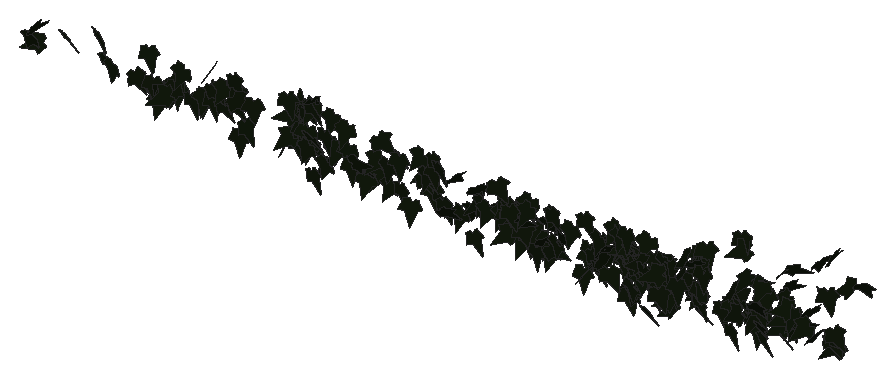
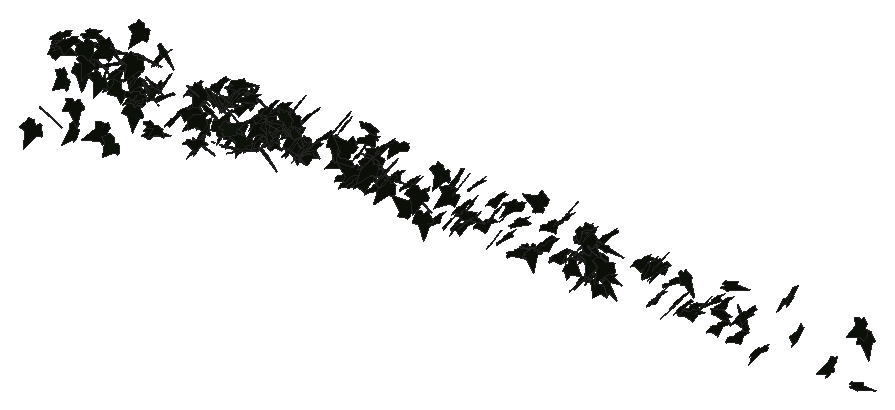
# SketchUp Ruby script. Lengths in inches.
U = 1.inch
M = Sketchup.active_model
def pt(a) = Geom::Point3d.new(a.map { |v| v * U })
def face(e, loops, mat)
  f = e.add_face(loops[0].map { |a| pt(a) })
  loops[1..].each { |l| e.add_face(l.map { |a| pt(a) }).erase! }
  f.material = f.back_material = mat if mat
  f
end
# faces: each face lists its corners as indices into pts; further lists are holes
def faces(e, pts, list, mat = nil) = list.each { |f| face(e, (f[0].is_a?(Array) ? f : [f]).map { |l| l.map { |i| pts[i] } }, mat) }
# xy, xz, yz: faces in a plane at the given z, y or x. An outline is a flat list of corners, or four numbers for a rectangle; further outlines are holes
def ring(l) = l.size == 4 ? [[l[0], l[1]], [l[2], l[1]], [l[2], l[3]], [l[0], l[3]]] : l.each_slice(2).to_a
def flat(e, list, mat, &to3) = list.each { |f| face(e, (f[0].is_a?(Array) ? f : [f]).map { |l| ring(l).map { |u, v| to3.(u, v) } }, mat) }
def xy(e, z, list, mat = nil) = flat(e, list, mat) { |x, y| [x, y, z] }
def xz(e, y, list, mat = nil) = flat(e, list, mat) { |x, z| [x, y, z] }
def yz(e, x, list, mat = nil) = flat(e, list, mat) { |y, z| [x, y, z] }
def lines(e, pts, list) = list.each { |a, b| e.add_line(pt(pts[a]), pt(pts[b])) }
# prism: a flat outline (further loops are holes) pulled along v
def prism(e, loops, v, mat = nil)
  f = face(e, loops, mat); d = Geom::Vector3d.new(v.map { |x| x * U })
  f.pushpull(f.normal.samedirection?(d) ? d.length : -d.length)
end
def box(e, o, s, mat = nil) = prism(e, [[o, [o[0] + s[0], o[1], o[2]], [o[0] + s[0], o[1] + s[1], o[2]], [o[0], o[1] + s[1], o[2]]]], [0, 0, s[2]], mat)
def at(x, y, z, deg = 0) = Geom::Transformation.translation(pt([x, y, z])) * Geom::Transformation.rotation(ORIGIN, Z_AXIS, deg.degrees)
def axes(o, x, y, z) = Geom::Transformation.new([*x, 0, *y, 0, *z, 0, *pt(o).to_a, 1])
def part(name) = M.definitions.add(name)
# library, detail: a bought-in or finely detailed component or shape, given as its bounding box
def library(name, o, s) = part(name).tap { |d| box(d.entities, o, s) }
def detail(e, o, s) = box(e.add_group.entities, o, s)
def put(e, d, t, mat = nil) = e.add_instance(d, t).tap { |i| i.material = mat if mat }
def group(e, t, mat = nil) = e.add_group.tap { |g| g.transformation = t; g.material = mat if mat }.entities
root = M.entities
M.materials.add("efeu1").color = [18, 25, 13]
c1 = part("ivyleaf_9")
p = [[1.54,2.16,1.25],[1.36,2.04,1.19],[-0.21,0.99,0.68],[-0.71,1.11,0.82],[-0.85,0.86,0.67],[-0.8,0.17,0.21],
  [-0.9,-0.01,0.1],[-0.67,-0.16,-0.02],[-0.08,-0.08,-0.05],[-0.03,-0.6,-0.4],[0.65,-0.88,-0.66],[0.83,-0.6,-0.49],
  [1.29,-0.42,-0.43],[1.8125,-0.07,-0.26],[1.21,0.44,0.15]]
faces(c1.entities,p,[[0,1,2,3,4,5,6,7,8,9,10,11,12,13,14]],"efeu1")
put(root,c1,axes([41.69,218.71,259.01],[0.16573,-0.44796,-0.14787],[-0.00628,0.15462,-0.47545],[0.47169,0.15945,0.04562]))
put(root,c1,axes([39.24,220.66,258.88],[-0.07317,-0.4717,0.14881],[-0.03935,-0.1444,-0.47707],[0.49305,-0.08153,-0.01599]))
put(root,c1,axes([54.97,220.37,258.9375],[0.15145,-0.468,-0.08964],[-0.03961,0.08137,-0.49174],[0.47486,0.15605,-0.01243]))
put(root,c1,axes([16.32,220.39,258.81],[-0.18161,-0.46555,0.01669],[-0.00257,-0.01691,-0.49971],[0.46584,-0.18159,0.00375]))
put(root,c1,axes([22.93,219.74,258.84],[0.01164,-0.49829,0.03967],[0.00611,-0.03954,-0.4984],[0.49983,0.01209,0.00516]))
put(root,c1,axes([39.71,221.03,259.17],[0.32737,0.18521,-0.32943],[-0.29143,-0.15376,-0.37607],[-0.24061,0.43824,0.00728]))
put(root,c1,axes([32.42,220.2,259.08],[-0.36225,-0.30732,-0.15597],[0.1342,0.08264,-0.47451],[0.31743,-0.38565,0.02261]))
put(root,c1,axes([29.26,220.11,259.07],[-0.14548,0.17352,-0.44579],[0.24229,-0.37503,-0.22505],[-0.41247,-0.2815,0.02503]))
put(root,c1,axes([61.79,221.22,258.85],[0.05915,0.49649,0.00142],[-0.00255,0.00173,-0.49999],[-0.49648,0.05915,0.00274]))
put(root,c1,axes([13.71,221.22,259.1875],[0.14882,-0.40431,-0.25374],[-0.02746,0.25809,-0.42736],[0.47655,0.14113,0.05461]))
put(root,c1,axes([26.28,221.05,259.14],[-0.25408,-0.11462,-0.4151],[0.37181,0.18476,-0.27861],[0.21726,-0.45025,-0.00866]))
put(root,c1,axes([32.18,220.24,259.23],[0.29071,0.15833,-0.37473],[-0.31652,-0.20129,-0.3306],[-0.25554,0.42944,-0.0168]))
put(root,c1,axes([62.04,220.71,258.93],[-0.07555,-0.49374,0.02259],[-0.00396,-0.02225,-0.49949],[0.49424,-0.07565,-0.00055]))
put(root,c1,axes([36.5,219.28,259.08],[-0.15881,-0.46494,-0.0928],[0.04255,0.08349,-0.49114],[0.4722,-0.16389,0.01305]))
put(root,c1,axes([52.36,220.61,258.96],[-0.42761,0.25803,-0.02383],[0.02061,-0.01196,-0.49943],[-0.25831,-0.42811,-0.00041]))
put(root,c1,axes([62.79,219.9,258.9375],[0.35697,-0.35001,-0.00792],[-0.00575,0.00545,-0.49994],[0.35005,0.35702,-0.00013]))
put(root,c1,axes([44.42,220.125,259.06],[-0.13816,-0.46076,0.13643],[-0.02366,-0.13526,-0.48078],[0.47995,-0.1393,0.01557]))
put(root,c1,axes([25.93,220.79,259.3],[-0.36566,0.2183,-0.26199],[0.20922,-0.15974,-0.4251],[-0.2693,-0.42051,0.02548]))
put(root,c1,axes([27.32,221.23,259.16],[0.30537,-0.38504,-0.09217],[0.01165,0.12509,-0.48396],[0.39574,0.29342,0.08537]))
put(root,c1,axes([54.62,219.83,259.08],[0.18919,-0.4047,0.22455],[0.1068,-0.19787,-0.44659],[0.45033,0.21695,0.01158]))
put(root,c1,axes([6.75,220.89,258.99],[-0.38467,-0.03692,0.25686],[-0.25164,-0.10565,-0.36589],[0.09703,-0.42036,0.0694]))
put(root,c1,axes([34.71,220.43,259.08],[0.2028,-0.45648,0.02225],[0.00841,-0.02061,-0.4995],[0.45695,0.20297,-0.00069]))
put(root,c1,axes([58.93,221,259.14],[0.08504,-0.49088,-0.04243],[-0.00119,0.04285,-0.49816],[0.49271,0.08483,0.00612]))
put(root,c1,axes([38.07,220.35,259.25],[0.19269,-0.4498,-0.10273],[-0.01302,0.10598,-0.48847],[0.4612,0.19092,0.02913]))
put(root,c1,axes([46.64,220.1,259.11],[-0.18728,-0.46245,0.03264],[-0.00218,-0.03432,-0.49882],[0.4636,-0.18698,0.01083]))
put(root,c1,axes([34.23,220.23,259.19],[-0.14658,-0.42022,0.22788],[-0.02607,-0.23097,-0.44269],[0.47732,-0.14166,0.0458]))
put(root,c1,axes([52.9,221.55,259.33],[0.24652,-0.36119,-0.24243],[0.20815,0.34262,-0.2988],[0.38197,0.04639,0.31929]))
put(root,c1,axes([53.79,218.56,259.38],[-0.02969,-0.46767,-0.17437],[0.04877,0.17112,-0.46727],[0.49673,-0.04475,0.03545]))
put(root,c1,axes([53.83,218.93,259.17],[-0.04068,-0.3651,0.33919],[0.10105,-0.33929,-0.35309],[0.48799,0.03982,0.10139]))
put(root,c1,axes([57.86,219.92,259.12],[0.48604,-0.11731,-0.00069],[-0.00037,0.00138,-0.5],[0.11731,0.48604,0.00125]))
put(root,c1,axes([32.71,221.06,259.17],[-0.31043,-0.38829,0.05349],[-0.0165,-0.05522,-0.49667],[0.39161,-0.31013,0.02147]))
put(root,c1,axes([29.59,219.73,259.24],[-0.09074,-0.41676,0.26091],[0.07648,-0.27405,-0.41115],[0.48571,-0.03471,0.11349]))
put(root,c1,axes([37.37,220.73,259.23],[0.21803,-0.43203,0.12574],[0.04934,-0.11592,-0.48387],[0.44724,0.22341,-0.00792]))
put(root,c1,axes([62.04,220.3,259.33],[0.4857,0.0514,-0.10701],[-0.10775,0.00161,-0.48825],[-0.04985,0.49735,0.01264]))
put(root,c1,axes([62.48,225.95,259.27],[0.47019,-0.16105,-0.0546],[-0.0544,0.00964,-0.49694],[0.16111,0.47326,-0.00846]))
put(root,c1,axes([53.09,220.74,259.22],[-0.10975,-0.48643,0.03663],[0.00253,-0.03811,-0.49854],[0.4878,-0.10924,0.01083]))
put(root,c1,axes([49.95,218.98,259.3125],[-0.02277,-0.4978,-0.0409],[-0.00504,0.04117,-0.49828],[0.49946,-0.02228,-0.0069]))
put(root,c1,axes([54.66,220.68,259.48],[-0.11745,-0.19356,-0.44581],[0.42836,0.17543,-0.18902],[0.22959,-0.42633,0.12462]))
put(root,c1,axes([45.78,220.8,259.31],[-0.12054,-0.481,0.06407],[-0.01894,-0.06131,-0.49587],[0.48488,-0.12197,-0.00344]))
put(root,c1,axes([53.82,220.59,259.36],[0.26998,0.41269,0.08248],[-0.12056,0.16973,-0.45459],[-0.40321,0.22557,0.19116]))
put(root,c1,axes([50.375,219.18,259.65],[-0.32192,0.25455,-0.2856],[0.12611,-0.2818,-0.3933],[-0.3612,-0.32526,0.11724]))
put(root,c1,axes([29.81,218.08,259.39],[0.23594,-0.43705,-0.05764],[-0.01788,0.05583,-0.49655],[0.44047,0.23637,0.01071]))
put(root,c1,axes([44.86,220.33,259.43],[-0.10661,-0.48137,-0.08319],[0.01205,0.08253,-0.49299],[0.48835,-0.10712,-0.006]))
put(root,c1,axes([59.57,226,259.39],[0.17712,0.35875,0.29987],[0.0105,0.31754,-0.38608],[-0.46746,0.14306,0.10495]))
put(root,c1,axes([27.34,220.94,259.375],[-0.08938,-0.48796,0.06251],[-0.00694,-0.06228,-0.49606],[0.4919,-0.08954,0.00435]))
put(root,c1,axes([56.33,220.95,259.5],[0.37584,-0.31786,-0.08783],[-0.07859,0.043,-0.49191],[0.32027,0.38356,-0.01764]))
put(root,c1,axes([54.625,220.75,259.67],[-0.35385,-0.25883,-0.24042],[0.20642,0.12466,-0.43801],[0.28668,-0.40923,0.01864]))
put(root,c1,axes([36.77,220.95,259.59],[-0.04253,-0.48051,-0.13152],[0.03312,0.12898,-0.48194],[0.49709,-0.04971,0.02086]))
put(root,c1,axes([64.37,227.57,259.56],[0.4073,0.27528,-0.09128],[-0.08776,-0.033,-0.49113],[-0.27642,0.41609,0.02143]))
put(root,c1,axes([45.16,220.92,259.51],[-0.23171,-0.38991,0.21044],[-0.06106,-0.20711,-0.45097],[0.43884,-0.23468,0.04837]))
put(root,c1,axes([20.5,220.95,259.66],[0.28001,-0.38775,-0.14576],[-0.00496,0.17278,-0.46917],[0.41421,0.26419,0.09292]))
put(root,c1,axes([49.34,220.45,259.64],[-0.26201,-0.40743,-0.1239],[0.13422,0.05906,-0.47801],[0.40415,-0.28375,0.07842]))
put(root,c1,axes([17.14,221.1,259.55],[-0.09752,-0.48565,-0.0681],[0.00461,0.06852,-0.49526],[0.49038,-0.09722,-0.00889]))
put(root,c1,axes([57.49,220.74,259.66],[0.0164,0.23513,-0.44096],[-0.30455,-0.34509,-0.19534],[-0.3962,0.275,0.1319]))
put(root,c1,axes([44,219.45,259.625],[-0.46706,-0.11291,0.13822],[-0.10279,-0.14639,-0.46691],[0.1459,-0.46457,0.11353]))
put(root,c1,axes([26.22,220.63,259.61],[-0.43913,-0.20773,0.11838],[-0.10836,-0.04776,-0.48577],[0.21313,-0.45229,-0.00307]))
put(root,c1,axes([19.25,221.02,259.75],[-0.23563,-0.42311,-0.12434],[0.10442,0.08344,-0.4818],[0.42846,-0.25302,0.04904]))
put(root,c1,axes([55.14,223.41,259.82],[0.32334,-0.33409,-0.18395],[-0.1165,0.14312,-0.4647],[0.36315,0.34337,0.0147]))
put(root,c1,axes([53.73,218.85,259.6875],[0.03024,-0.43514,0.24441],[0.13468,-0.22866,-0.42376],[0.48057,0.09146,0.10339]))
put(root,c1,axes([61.77,220.61,259.67],[-0.12781,-0.43897,0.20241],[-0.01881,-0.20469,-0.45579],[0.48302,-0.12413,0.03581]))
put(root,c1,axes([40.8125,220.99,259.07],[-0.02306,-0.1513,0.476],[0.48172,0.11917,0.06122],[-0.13198,0.46142,0.14027]))
put(root,c1,axes([57.32,218.41,259.64],[-0.43004,0.24718,0.06301],[-0.06249,0.01766,-0.49577],[-0.24731,-0.43427,0.0157]))
put(root,c1,axes([61.49,218.55,259.6],[0.26354,-0.42484,-0.00764],[-0.00427,0.00634,-0.49994],[0.42489,0.26357,-0.00028]))
put(root,c1,axes([55.35,223.22,259.73],[-0.49372,0.05722,-0.05448],[0.03949,-0.11994,-0.48379],[-0.06843,-0.48202,0.11392]))
put(root,c1,axes([55.05,223.31,259.67],[0.34376,-0.36173,-0.03131],[-0.02145,0.02281,-0.49902],[0.36245,0.34443,0.00016]))
put(root,c1,axes([63.98,219.98,259.63],[0.47281,-0.16259,0.00317],[0.00295,-0.00116,-0.49999],[0.1626,0.47282,-0.00013]))
put(root,c1,axes([61.97,221.16,259.81],[-0.40378,-0.27697,-0.10123],[0.09063,0.04678,-0.48949],[0.28062,-0.41364,0.01243]))
put(root,c1,axes([26.39,221.14,259.87],[0.18887,-0.44638,-0.12277],[0.03426,0.14571,-0.47707],[0.46169,0.1718,0.08563]))
put(root,c1,axes([50.34,220.68,259.75],[-0.49796,-0.01225,-0.04345],[0.04452,-0.05357,-0.49512],[0.00748,-0.49697,0.05444]))
put(root,c1,axes([58.09,219.83,259.73],[0.22386,-0.43493,0.10354],[0.07699,-0.07657,-0.48807],[0.44041,0.23446,0.03269]))
put(root,c1,axes([50.67,219.66,259.94],[0.07987,0.45465,-0.19212],[-0.01344,-0.19254,-0.46124],[-0.4934,0.07884,-0.01854]))
put(root,c1,axes([44.51,219.96,259.99],[-0.06521,-0.42857,-0.24915],[0.08718,0.23747,-0.43129],[0.488,-0.09969,0.04375]))
put(root,c1,axes([56.15,216.97,259.72],[0.4921,-0.08064,-0.03659],[-0.03581,0.00769,-0.49866],[0.08098,0.49339,0.00179]))
put(root,c1,axes([49.64,220.14,259.96],[0.24301,-0.38787,-0.20126],[-0.06196,0.19738,-0.4552],[0.43256,0.24617,0.04787]))
put(root,c1,axes([64.68,220.83,259.78],[0.10046,0.44382,0.2072],[-0.00703,0.21279,-0.4524],[-0.48975,0.08798,0.04899]))
put(root,c1,axes([66.26,220.6,259.74],[0.00095,0.49427,0.07544],[-0.02655,0.07539,-0.49357],[-0.49929,-0.00307,0.02639]))
put(root,c1,axes([39.33,218.67,259.78],[0.43694,0.19508,0.14501],[0.12825,0.06837,-0.47841],[-0.20649,0.45527,0.00971]))
put(root,c1,axes([51.6,220.92,260.0625],[-0.29164,-0.26929,-0.30402],[0.31034,0.09366,-0.38068],[0.26198,-0.41074,0.11251]))
put(root,c1,axes([45.79,219.95,259.22],[0.23112,0.43493,-0.08614],[0.03892,0.07686,0.49252],[0.44167,-0.23437,0.00167]))
put(root,c1,axes([31.37,219.88,259.79],[0.01229,-0.49841,-0.03791],[-0.01208,0.03761,-0.49844],[0.4997,0.01317,-0.01112]))
put(root,c1,axes([19.9,220.87,259.83],[0.07931,-0.4908,-0.05311],[0.00582,0.05471,-0.49696],[0.49364,0.07821,0.01439]))
put(root,c1,axes([52.03,218.82,260.1],[-0.09216,-0.34578,-0.3492],[0.25334,0.27101,-0.33522],[0.4211,-0.23872,0.12525]))
put(root,c1,axes([52.65,220.52,259.99],[0.19306,-0.42504,-0.17909],[-0.07474,0.16274,-0.46683],[0.45513,0.20702,-0.0007]))
put(root,c1,axes([55.03,220.82,260.07],[0.41335,-0.12484,-0.2521],[-0.23994,0.07744,-0.43178],[0.14685,0.47793,0.00411]))
put(root,c1,axes([16.01,219.78,259.26],[-0.06461,0.13814,0.47618],[0.21119,-0.4268,0.15247],[0.44858,0.22082,-0.0032]))
put(root,c1,axes([28.2,219.74,259.89],[-0.1261,-0.42195,0.23677],[0.03539,-0.25207,-0.43036],[0.48254,-0.09177,0.09344]))
put(root,c1,axes([64.54,220.8,259.7],[0.21885,-0.16164,-0.41949],[0.3376,-0.249,0.27208],[-0.29687,-0.40233,0.00015]))
put(root,c1,axes([57.28,218.625,259.81],[-0.37005,-0.02777,0.3351],[-0.33428,-0.02356,-0.37109],[0.0364,-0.49867,-0.00113]))
put(root,c1,axes([60.1875,225.96,259.87],[0.37223,0.12545,0.30937],[0.27404,0.14981,-0.39046],[-0.19066,0.46024,0.04277]))
put(root,c1,axes([47.0625,219.36,259.72],[0.02745,-0.04723,-0.49701],[0.25411,0.42978,-0.02681],[0.42974,-0.25112,0.0476]))
put(root,c1,axes([29.61,220.83,259.87],[-0.20986,-0.45033,0.0562],[-0.01511,-0.05496,-0.49674],[0.45357,-0.21019,0.00946]))
put(root,c1,axes([50.8,219.12,259.88],[0.30972,-0.38753,0.06243],[0.04191,-0.04642,-0.49607],[0.39028,0.31252,0.00372]))
put(root,c1,axes([46.73,218.42,259.9],[0.09436,-0.48341,0.08611],[0.00691,-0.08637,-0.49243],[0.49097,0.09412,-0.00962]))
put(root,c1,axes([53.77,221.72,259.18],[0.4983,-0.0009,-0.04115],[0.0028,0.49946,0.02305],[0.04107,-0.0232,0.49777]))
put(root,c1,axes([64.3,220.29,259.88],[-0.26768,-0.21714,0.36221],[-0.16084,-0.34411,-0.32515],[0.39049,-0.29058,0.11437]))
put(root,c1,axes([36.2,220.7,260.14],[0.2277,-0.41442,-0.16251],[0.04668,0.20377,-0.4542],[0.44269,0.19167,0.13149]))
put(root,c1,axes([60.08,220.6,260.07],[-0.0337,-0.48837,-0.1018],[0.16746,0.08504,-0.46339],[0.46992,-0.06532,0.15783]))
put(root,c1,axes([19.41,220.86,259.89],[-0.16168,-0.47281,0.01758],[0.00196,-0.01925,-0.49963],[0.47313,-0.16149,0.00807]))
put(root,c1,axes([8.19,221.2,259.95],[0.39839,-0.28631,0.09649],[0.09239,-0.03658,-0.49003],[0.28766,0.40828,0.02376]))
put(root,c1,axes([63.02,221.01,259.71],[-0.20239,0.32814,-0.31837],[-0.16632,0.27147,0.38554],[0.42588,0.26196,-0.00073]))
put(root,c1,axes([18.95,220.03,259.93],[0.17931,-0.46594,-0.02736],[-0.00666,0.02675,-0.49924],[0.46669,0.1794,0.00339]))
put(root,c1,axes([21.58,220.74,260.17],[0.3021,-0.35458,-0.18168],[-0.0486,0.1935,-0.45847],[0.39544,0.29467,0.08245]))
put(root,c1,axes([64.5625,226.38,260],[-0.40796,0.24106,0.15954],[-0.16255,0.03689,-0.4714],[-0.23905,-0.43649,0.04827]))
put(root,c1,axes([16.05,220.02,260.04],[-0.03343,-0.49333,-0.07424],[0.04361,0.07123,-0.49297],[0.49697,-0.03944,0.03827]))
put(root,c1,axes([49.15,220.48,260.01],[0.10157,-0.47537,0.11709],[0.02379,-0.11465,-0.4861],[0.489,0.10432,-0.00067]))
put(root,c1,axes([54.98,224,260.24],[-0.24806,-0.39153,-0.18753],[0.15276,0.12345,-0.45981],[0.40636,-0.28542,0.05837]))
put(root,c1,axes([61.7,220.19,260.07],[-0.40651,0.28662,-0.05099],[0.04639,-0.02269,-0.49733],[-0.2874,-0.40907,-0.00815]))
put(root,c1,axes([42.78,220.54,260.02],[0.45585,0.20495,-0.01394],[-0.0132,-0.00465,-0.4998],[-0.205,0.45604,0.00117]))
put(root,c1,axes([47.375,219.625,260.12],[0.03099,-0.42769,0.25714],[0.08492,-0.24935,-0.42498],[0.49176,0.07002,0.05718]))
put(root,c1,axes([29.41,220.93,260.09],[-0.10067,-0.48783,-0.04342],[0.00299,0.04371,-0.49808],[0.48975,-0.10054,-0.00588]))
put(root,c1,axes([57.97,220.22,260.14],[-0.19334,-0.40555,0.21943],[-0.05572,-0.21564,-0.44765],[0.45773,-0.19755,0.03819]))
put(root,c1,axes([17.52,220.52,260.15],[-0.46793,-0.16429,-0.06364],[0.05728,0.02891,-0.49587],[0.16661,-0.47135,-0.00824]))
put(root,c1,axes([40.67,220.59,260.09],[-0.47129,0.16676,-0.0086],[0.00526,-0.01092,-0.49985],[-0.1669,-0.47125,0.00853]))
put(root,c1,axes([51.83,220.65,260.125],[-0.02083,-0.49478,0.06899],[-0.00624,-0.06879,-0.49521],[0.49953,-0.0215,-0.0033]))
put(root,c1,axes([51.68,220.59,260.26],[0.41021,-0.27013,-0.09357],[-0.05755,0.08227,-0.48982],[0.28002,0.41263,0.0364]))
put(root,c1,axes([60.48,220.84,260.21],[0.16317,-0.39212,0.26386],[0.20734,-0.19146,-0.41274],[0.42472,0.24411,0.10012]))
put(root,c1,axes([51.87,220.72,260.43],[-0.39124,-0.14506,-0.27548],[0.26218,0.08508,-0.41716],[0.16791,-0.47087,0.00949]))
put(root,c1,axes([24.09,218.8125,260.4],[0.15106,-0.43018,-0.20525],[-0.05931,0.19668,-0.45585],[0.47293,0.16207,0.00839]))
put(root,c1,axes([62.14,220.65,260.5],[-0.1874,-0.32625,-0.3293],[0.23879,0.2365,-0.3702],[0.39732,-0.29602,0.06717]))
put(root,c1,axes([41.72,220.11,260.25],[-0.12547,-0.45523,0.16438],[-0.01502,-0.16607,-0.47138],[0.48377,-0.12323,0.028]))
put(root,c1,axes([42.92,220.35,260.2],[-0.01585,-0.49946,-0.01711],[-0.01839,0.01769,-0.49935],[0.49941,-0.0152,-0.01893]))
put(root,c1,axes([26.71,220.95,260.23],[0.02157,-0.49923,-0.01738],[-0.00001,0.01739,-0.4997],[0.49953,0.02156,0.00074]))
put(root,c1,axes([30.59,220.68,260.23],[-0.06932,-0.49413,0.03215],[-0.00061,-0.03238,-0.49895],[0.49517,-0.06922,0.00389]))
put(root,c1,axes([41.18,220.27,260.31],[-0.09723,-0.38036,0.30963],[0.04521,-0.32126,-0.38046],[0.48837,-0.04599,0.09687]))
put(root,c1,axes([17.79,219.88,260.3125],[-0.07559,-0.48802,0.07822],[-0.02242,-0.07566,-0.49373],[0.49374,-0.07815,-0.01044]))
put(root,c1,axes([27.84,220.15,260.37],[0.34932,-0.34476,0.09546],[0.14109,0.01017,-0.47957],[0.32874,0.36199,0.10439]))
put(root,c1,axes([57.79,220.3,260.3],[0.02981,-0.49825,0.02928],[-0.00586,-0.02968,-0.49908],[0.49908,0.02942,-0.00761]))
put(root,c1,axes([19.86,220.84,260.6],[0.26088,-0.36655,-0.21813],[-0.02031,0.24473,-0.43554],[0.42606,0.23611,0.1128]))
put(root,c1,axes([42.82,220.22,260.41],[-0.16322,-0.46023,0.10746],[-0.02535,-0.105,-0.48819],[0.47193,-0.16482,0.01094]))
put(root,c1,axes([68.67,220.11,260.21],[-0.0373,-0.01631,-0.49834],[-0.04251,-0.49781,0.01947],[-0.49679,0.04383,0.03575]))
put(root,c1,axes([65.94,220.17,260.41],[0.22563,0.44222,0.05942],[0.03132,0.05073,-0.49643],[-0.44509,0.22775,-0.00481]))
put(root,c1,axes([51.51,219.33,260.1],[-0.38339,0.21841,-0.23517],[-0.20376,0.11742,0.44124],[0.24797,0.43418,-0.00103]))
put(root,c1,axes([68.2,220,260.71],[0.05281,-0.42555,-0.25714],[0.04577,0.26164,-0.42361],[0.49509,0.0212,0.06659]))
put(root,c1,axes([56.57,217.88,260.72],[-0.15218,-0.33177,-0.34171],[0.2058,0.27771,-0.36128],[0.42952,-0.25061,0.05203]))
put(root,c1,axes([36.45,221.19,260.46],[-0.44486,-0.14425,0.1769],[-0.1682,-0.05481,-0.46766],[0.15432,-0.47559,0.00024]))
put(root,c1,axes([27.6,220.42,260.56],[-0.20618,-0.44594,-0.09289],[0.1083,0.05105,-0.48545],[0.44245,-0.2203,0.07554]))
put(root,c1,axes([56.83,220.62,260.4375],[-0.4958,0.06197,0.01858],[-0.01939,-0.00531,-0.4996],[-0.06173,-0.49612,0.00767]))
put(root,c1,axes([49.62,221.19,260.51],[0.30168,-0.39805,-0.02331],[-0.00013,0.02913,-0.49915],[0.39874,0.30117,0.01747]))
put(root,c1,axes([64.49,220.42,260.58],[-0.40414,-0.15086,0.25281],[-0.1434,-0.27411,-0.39281],[0.25711,-0.39,0.1783]))
put(root,c1,axes([50.92,221.04,260.67],[0.35232,-0.34508,-0.08239],[0.02418,0.1392,-0.47962],[0.35395,0.33398,0.11477]))
put(root,c1,axes([57.4375,225.39,260.5625],[-0.37642,-0.1329,0.30107],[-0.26903,-0.13919,-0.39781],[0.18955,-0.46148,0.03328]))
put(root,c1,axes([53.17,220.02,260.83],[0.03272,-0.42127,-0.26733],[-0.02806,0.26592,-0.42249],[0.49814,0.04265,-0.00623]))
put(root,c1,axes([18.59,218.34,260.62],[-0.40367,-0.13443,0.26263],[-0.2316,-0.13136,-0.42321],[0.18279,-0.46333,0.04379]))
put(root,c1,axes([33.22,220.28,260.65],[-0.2737,-0.37267,0.19028],[-0.07164,-0.18228,-0.46005],[0.41226,-0.27909,0.04638]))
put(root,c1,axes([44.68,219.13,260.63],[0.3405,0.25433,0.26339],[0.20641,0.16375,-0.42495],[-0.30241,0.39813,0.00652]))
put(root,c1,axes([34.21,219.87,260.6875],[0.0084,-0.44565,0.22655],[0.0696,-0.22333,-0.4419],[0.49506,0.03896,0.05829]))
put(root,c1,axes([36.63,220.5625,260.67],[0.01287,-0.44347,0.23059],[-0.00469,-0.23077,-0.44354],[0.49981,0.00926,-0.0101]))
put(root,c1,axes([40.13,220.92,260.65],[0.2468,0.43254,-0.04474],[-0.01994,-0.04013,-0.49799],[-0.43439,0.24759,-0.00256]))
put(root,c1,axes([51.96,220.375,260.68],[-0.02057,0.47814,0.14476],[-0.03846,0.14294,-0.47759],[-0.49809,-0.03078,0.0309]))
put(root,c1,axes([47.92,219.375,260.87],[0.26375,0.0668,-0.41949],[-0.4184,-0.04438,-0.27013],[-0.07333,0.49353,0.03249]))
put(root,c1,axes([51.21,218.93,260.52],[0.00466,0.09511,-0.49085],[-0.21308,0.44444,0.08409],[0.4523,0.20839,0.04468]))
put(root,c1,axes([7.83,218.39,260.94],[0.28455,0.13928,-0.38682],[-0.36268,-0.13651,-0.31595],[-0.19363,0.4604,0.02334]))
put(root,c1,axes([55.84,218.97,260.65],[0.04123,-0.49788,0.02032],[0.00326,-0.02012,-0.49958],[0.49829,0.04132,0.00159]))
put(root,c1,axes([65.2,220.55,260.76],[-0.48215,0.11354,-0.06813],[0.0612,-0.03706,-0.49486],[-0.11742,-0.48553,0.02184]))
put(root,c1,axes([54.9375,221.78,260.1],[-0.45794,-0.08004,0.18407],[0.10732,-0.48512,0.05606],[0.16962,0.09086,0.46149]))
put(root,c1,axes([25.74,220.83,260.73],[0.33446,0.36565,0.06664],[0.03702,0.05643,-0.49542],[-0.36982,0.33633,0.01067]))
put(root,c1,axes([43.03,220.34,260.95],[0.25598,-0.39825,-0.16085],[-0.05473,0.15548,-0.47205],[0.426,0.25928,0.03601]))
put(root,c1,axes([50.46,220.04,260.78],[-0.33907,0.36624,-0.02998],[0.02181,-0.02066,-0.4991],[-0.36681,-0.33977,-0.00197]))
put(root,c1,axes([27.01,220.92,260.79],[-0.04354,0.49041,0.08716],[-0.0065,0.08693,-0.49234],[-0.49806,-0.04401,-0.00119]))
put(root,c1,axes([55.64,220.14,260.79],[0.0177,-0.38179,0.32237],[0.07493,-0.3169,-0.37942],[0.49404,0.06174,0.046]))
put(root,c1,axes([52.5,220.48,260.53],[-0.18732,0.07902,0.4568],[-0.46357,-0.03602,-0.18387],[0.00385,-0.4924,0.08676]))
put(root,c1,axes([54.25,221.93,260.4],[-0.49768,-0.03916,0.02793],[0.02617,-0.46407,-0.18426],[0.04036,-0.18195,0.46397]))
put(root,c1,axes([52.13,220.51,260.87],[0.32222,-0.35988,0.12906],[0.13672,-0.04916,-0.47842],[0.35704,0.34361,0.06673]))
put(root,c1,axes([26.68,220.88,260.86],[0.18304,0.44868,0.12323],[0.00506,0.1305,-0.48264],[-0.46527,0.17793,0.04323]))
put(root,c1,axes([56.63,220.2,261.07],[-0.39324,0.26034,-0.16608],[0.09195,-0.15798,-0.46539],[-0.2948,-0.39656,0.07637]))
put(root,c1,axes([36.77,221.05,260.89],[0.02474,-0.49641,-0.05448],[-0.00317,0.05439,-0.49702],[0.49938,0.02494,-0.00046]))
put(root,c1,axes([68.37,219.98,261.18],[0.05613,-0.41138,-0.27859],[0.05278,0.28372,-0.40831],[0.49403,0.01643,0.07527]))
put(root,c1,axes([52.92,220,260.98],[0.42414,-0.24937,-0.08902],[-0.06905,0.05812,-0.49179],[0.25562,0.42946,0.01486]))
put(root,c1,axes([61.76,221.08,260.92],[0.19182,-0.40771,0.21675],[0.08759,-0.19832,-0.45055],[0.45336,0.21082,-0.00466]))
put(root,c1,axes([17.71,220.85,260.95],[-0.17022,-0.43606,0.17572],[-0.00641,-0.18471,-0.46459],[0.47009,-0.16041,0.05729]))
put(root,c1,axes([44.125,220.5,260.89],[0.47478,0.15347,-0.03217],[-0.03116,-0.0082,-0.49896],[-0.15368,0.47579,0.00178]))
put(root,c1,axes([34.55,220.61,260.94],[0.05787,-0.43645,0.23698],[0.07293,-0.22853,-0.4387],[0.49126,0.08534,0.03721]))
put(root,c1,axes([10.94,221.04,261],[0.26285,-0.37522,0.20029],[0.10006,-0.1743,-0.45783],[0.4134,0.28076,-0.01654]))
put(root,c1,axes([62.24,218.58,260.8125],[-0.17314,-0.21107,0.41889],[-0.15115,-0.39759,-0.26282],[0.44405,-0.21764,0.07387]))
put(root,c1,axes([60.85,220.57,260.52],[-0.457,0.13393,-0.15237],[-0.1466,0.04155,0.47622],[0.14022,0.47994,0.00129]))
put(root,c1,axes([21.03,220.72,261.03],[-0.22925,-0.41521,0.15827],[0.00145,-0.17879,-0.46694],[0.44435,-0.21363,0.08318]))
put(root,c1,axes([14.0625,218.56,261],[0.04213,-0.4071,0.28721],[0.08819,-0.27759,-0.4064],[0.49035,0.0849,0.04841]))
put(root,c1,axes([56.84,225.52,261.27],[-0.23043,-0.20227,-0.39495],[0.33987,0.20566,-0.30362],[0.28528,-0.4084,0.04271]))
put(root,c1,axes([52.17,220.75,260.99],[0.4968,0.03221,0.04642],[0.04608,0.00678,-0.49783],[-0.0327,0.49892,0.00377]))
put(root,c1,axes([52.29,220.41,261.07],[-0.4094,-0.04244,0.28388],[-0.26782,-0.12143,-0.40439],[0.10327,-0.48317,0.0767]))
put(root,c1,axes([51.27,219.03,261.0625],[0.22475,0.4255,0.13579],[0.06725,0.11805,-0.48119],[-0.44155,0.23455,-0.00417]))
put(root,c1,axes([42.92,220.1,261],[0.19403,-0.46036,0.02048],[0.00809,-0.01881,-0.49958],[0.46075,0.1942,0.00015]))
put(root,c1,axes([46.32,219.91,260.76],[0.08213,-0.19444,0.45326],[0.42395,-0.20698,-0.16561],[0.25203,0.41152,0.13087]))
put(root,c1,axes([57.3,218.79,261.14],[-0.03943,-0.494,-0.06637],[-0.00654,0.06709,-0.49544],[0.4984,-0.0382,-0.01176]))
put(root,c1,axes([62.45,226.15,261.17],[0.00004,0.49297,-0.08356],[-0.00355,-0.08356,-0.49296],[-0.49999,0.00063,0.00349]))
put(root,c1,axes([54.21,220.33,261.26],[-0.03522,-0.48444,-0.11866],[0.07294,0.11268,-0.48165],[0.4934,-0.05123,0.06274]))
put(root,c1,axes([23.8125,219.97,261.23],[-0.0948,-0.47777,-0.1129],[0.0153,0.11206,-0.48704],[0.49069,-0.0958,-0.00662]))
put(root,c1,axes([55.99,219.94,261.13],[-0.49149,0.08836,-0.02515],[0.01429,-0.0617,-0.49597],[-0.09076,-0.48825,0.05813]))
put(root,c1,axes([14.91,221.04,261.28],[0.00331,-0.48067,-0.13764],[0.00606,0.13767,-0.48064],[0.49995,0.00151,0.00674]))
put(root,c1,axes([65.17,220.05,261.41],[-0.38969,-0.19865,-0.24225],[0.24038,0.05835,-0.43453],[0.20091,-0.45512,0.05002]))
put(root,c1,axes([48.22,220.01,261.2],[-0.0989,-0.4768,0.11348],[0.0441,-0.12395,-0.48238],[0.48813,-0.0854,0.06657]))
put(root,c1,axes([22.02,220.63,261.3],[0.14749,-0.46572,-0.10654],[0.02596,0.11915,-0.4849],[0.47705,0.1375,0.05932]))
put(root,c1,axes([44.1,220.45,261.36],[0.23988,-0.41534,-0.14125],[-0.00502,0.15838,-0.47423],[0.43867,0.22894,0.07182]))
put(root,c1,axes([62.51,220.82,261.39],[-0.22744,-0.40329,-0.18876],[0.10139,0.15949,-0.46291],[0.43358,-0.24885,0.00923]))
put(root,c1,axes([22.58,219.66,261.28],[0.06012,-0.15869,-0.47032],[0.02401,0.47414,-0.15691],[0.49579,-0.00372,0.06463]))
put(root,c1,axes([56.25,222.88,261.46],[-0.1296,-0.42113,-0.23633],[0.13138,0.20471,-0.43684],[0.4647,-0.17533,0.05759]))
put(root,c1,axes([54.58,218.9,261.23],[0.23382,-0.43521,0.07698],[0.03958,-0.06612,-0.49403],[0.44019,0.23712,0.00353]))
put(root,c1,axes([26.64,220.27,261.29],[-0.42488,0.09354,0.24642],[-0.25243,-0.00989,-0.43149],[-0.07585,-0.49107,0.05563]))
put(root,c1,axes([54.42,218.99,261.33],[-0.3694,0.29767,0.15792],[-0.20075,-0.0062,-0.45789],[-0.27064,-0.40169,0.1241]))
put(root,c1,axes([66.13,220.6,261.54],[-0.12538,0.42919,-0.22377],[-0.0067,-0.23267,-0.44252],[-0.48398,-0.10797,0.06409]))
put(root,c1,axes([32.92,218.16,261.02],[0.17486,-0.07496,0.46239],[0.41634,-0.20132,-0.19008],[0.21468,0.4515,-0.00799]))
put(root,c1,axes([55.04,220.24,261.39],[0.11843,-0.43843,0.20918],[0.09259,-0.19099,-0.45272],[0.47687,0.14597,0.03595]))
put(root,c1,axes([57.72,220.7,261.41],[-0.36955,0.30698,0.13854],[-0.17636,-0.00116,-0.46786],[-0.28693,-0.39467,0.10914]))
put(root,c1,axes([66.98,219.22,261.375],[-0.40539,-0.2481,0.15527],[-0.1269,-0.09004,-0.47517],[0.26374,-0.42466,0.01003]))
put(root,c1,axes([56.14,218.64,261.33],[-0.33343,-0.12388,0.35139],[-0.31208,-0.16474,-0.35421],[0.20354,-0.45554,0.03253]))
put(root,c1,axes([64.95,220.04,261.39],[-0.39419,0.02057,0.30691],[-0.30742,-0.04337,-0.39193],[0.0105,-0.49769,0.04684]))
put(root,c1,axes([44.24,218.98,261.56],[0.08221,-0.47179,-0.14373],[0.01654,0.14827,-0.47722],[0.49292,0.07371,0.03998]))
put(root,c1,axes([44.45,220.47,261.375],[-0.49927,-0.01868,-0.01956],[0.02077,-0.03332,-0.49846],[0.01731,-0.49854,0.03404]))
put(root,c1,axes([35.11,219.83,261.47],[-0.03293,-0.49524,-0.06045],[0.00856,0.06001,-0.49631],[0.49884,-0.03372,0.00452]))
put(root,c1,axes([57.85,220.53,261.38],[0.02845,-0.49918,0.00265],[-0.00004,-0.00266,-0.49999],[0.49919,0.02845,-0.00019]))
put(root,c1,axes([8,218.38,261.39],[0.20967,0.2336,0.38919],[0.17149,0.35616,-0.30616],[-0.42027,0.26188,0.06924]))
put(root,c1,axes([57.03,220.68,261.5625],[0.35683,0.34316,-0.07013],[-0.05893,-0.03987,-0.49491],[-0.34526,0.36146,0.01199]))
put(root,c1,axes([39.43,219.51,261.6875],[0.1946,0.43256,0.1582],[0.0243,0.16186,-0.47245],[-0.45994,0.19156,0.04197]))
put(root,c1,axes([13.625,218.2,261.61],[0.35796,-0.34894,-0.01026],[-0.00798,0.00652,-0.49989],[0.349,0.35805,-0.0009]))
put(root,c1,axes([30.47,220.625,261.63],[-0.23986,-0.43871,0.00102],[-0.00466,0.00138,-0.49998],[0.43869,-0.23986,-0.00475]))
put(root,c1,axes([51.17,220.01,261.67],[-0.21551,0.44984,0.03469],[-0.01584,0.03088,-0.49879],[-0.45089,-0.21609,0.00094]))
put(root,c1,axes([33.2,220.29,261.98],[0.07794,-0.28132,-0.40594],[0.06391,0.41325,-0.27411],[0.48974,-0.00916,0.10038]))
put(root,c1,axes([56.4,220.74,261.7],[-0.39704,0.30386,0.00497],[0.0049,0.01457,-0.49976],[-0.30386,-0.39681,-0.01455]))
put(root,c1,axes([20,220.62,261.85],[-0.26835,0.40942,-0.10181],[0.05984,-0.0825,-0.4895],[-0.41762,-0.2749,-0.00472]))
put(root,c1,axes([26.48,220.95,261.11],[-0.47566,0.15278,-0.02013],[-0.01845,0.00837,0.49959],[0.15299,0.47601,-0.00232]))
put(root,c1,axes([64.46,220.49,261.88],[-0.4902,-0.0311,-0.09348],[0.09402,-0.00608,-0.49104],[0.02941,-0.49899,0.01181]))
put(root,c1,axes([27.34,220.37,262.08],[0.26062,-0.32305,-0.27877],[-0.12121,0.25715,-0.41131],[0.40913,0.28197,0.05572]))
put(root,c1,axes([51.04,219.1,261.85],[-0.02187,-0.42439,0.26347],[0.01625,-0.26419,-0.42419],[0.49926,-0.00999,0.02535]))
put(root,c1,axes([51.67,220.47,261.86],[-0.09445,-0.47798,0.11232],[0.01374,-0.11691,-0.48595],[0.49081,-0.08871,0.03522]))
put(root,c1,axes([27.31,220.76,261.98],[0.11722,0.47361,-0.10932],[-0.01564,-0.10872,-0.48779],[-0.48581,0.11778,-0.01068]))
put(root,c1,axes([47.12,219.55,261.9],[-0.0455,-0.37654,0.3258],[0.04314,-0.32891,-0.37411],[0.49605,-0.00593,0.06242]))
put(root,c1,axes([37.23,220.33,262.07],[0.27062,-0.40081,-0.12696],[-0.05347,0.11695,-0.48318],[0.41702,0.27509,0.02044]))
put(root,c1,axes([36.53,220.2,261.98],[-0.19135,-0.37121,0.27494],[-0.02824,-0.28764,-0.408],[0.46107,-0.17167,0.08911]))
put(root,c1,axes([61.98,220.78,261.92],[0.37347,0.33242,0.00427],[-0.03449,0.04513,-0.49676],[-0.33066,0.37076,0.05663]))
put(root,c1,axes([62.42,220.64,262.07],[-0.40885,-0.26896,-0.1025],[0.09652,0.03963,-0.48899],[0.27116,-0.41963,0.01952]))
put(root,c1,axes([37.9375,219.89,261.94],[0.31007,-0.39017,0.04028],[0.01664,-0.03822,-0.49826],[0.3919,0.31033,-0.01072]))
put(root,c1,axes([30.22,218.76,261.92],[0.16485,-0.4718,0.01523],[-0.00081,-0.01642,-0.49973],[0.47204,0.16474,-0.00618]))
put(root,c1,axes([27.72,220.875,262.05],[-0.23668,-0.42021,0.13192],[0.00255,-0.15107,-0.47662],[0.44043,-0.22494,0.07366]))
put(root,c1,axes([21.91,220.41,262.11],[0.21527,-0.44386,-0.0815],[-0.00579,0.08757,-0.49224],[0.45125,0.21287,0.03257]))
put(root,c1,axes([66.35,221.9,262.27],[-0.08888,-0.43772,-0.22472],[0.05285,0.21854,-0.44659],[0.48919,-0.10314,0.00741]))
put(root,c1,axes([61.33,220.64,262.21],[-0.46889,-0.11282,-0.13197],[0.16456,-0.16759,-0.4414],[0.05537,-0.45737,0.19429]))
put(root,c1,axes([52.04,220.49,262.03],[0.04017,-0.49621,0.04649],[-0.01027,-0.04745,-0.49764],[0.49828,0.03903,-0.014]))
put(root,c1,axes([61.5625,218.89,262.09],[-0.38127,0.32115,-0.03867],[0.03928,-0.01337,-0.49828],[-0.32108,-0.38299,-0.01503]))
put(root,c1,axes([27.63,220.74,262.36],[-0.13963,0.34856,-0.33016],[0.07955,-0.32229,-0.3739],[-0.47347,-0.15695,0.03455]))
put(root,c1,axes([27.6,220.62,262.1875],[0.25148,-0.42834,-0.0573],[0.04263,0.09056,-0.48988],[0.43005,0.24151,0.08207]))
put(root,c1,axes([53.77,220.51,262.13],[-0.2857,-0.407,0.05221],[0.01045,-0.07081,-0.49485],[0.4102,-0.28167,0.04897]))
put(root,c1,axes([29.6,220.4,262.1875],[-0.13221,-0.46114,0.14097],[0.04454,-0.15723,-0.47254],[0.48014,-0.1124,0.08265]))
put(root,c1,axes([45.93,218.78,262.24],[-0.47548,-0.11128,-0.1074],[0.10254,0.0331,-0.48825],[0.11578,-0.48633,-0.00865]))
put(root,c1,axes([45.16,219.86,262.08],[-0.30592,-0.3953,0.01221],[-0.0025,-0.0135,-0.49981],[0.39548,-0.30587,0.00628]))
put(root,c1,axes([51.4375,220.38,262.18],[-0.25529,-0.40767,0.13652],[-0.0484,-0.13051,-0.48023],[0.42718,-0.25841,0.02718]))
put(root,c1,axes([63.79,225.35,262.07],[0.10793,0.30238,0.3833],[0.09172,0.373,-0.32009],[-0.47952,0.13941,0.02505]))
put(root,c1,axes([49.25,219.91,262.34],[0.16034,-0.45274,-0.139],[0.02749,0.1554,-0.47444],[0.4728,0.1445,0.07472]))
put(root,c1,axes([63.91,220.96,262.17],[0.27791,0.27862,0.30844],[0.20268,0.23309,-0.39318],[-0.36288,0.34357,0.01662]))
put(root,c1,axes([26.13,220.3,262.33],[0.03442,-0.4823,-0.12728],[0.04687,0.13014,-0.48049],[0.49661,0.02115,0.05417]))
put(root,c1,axes([42.67,219.72,262.47],[-0.03172,-0.34458,-0.36092],[0.11068,0.34778,-0.34176],[0.48656,-0.10157,0.05421]))
put(root,c1,axes([47.29,219.1875,262.34],[0.24618,-0.41285,-0.13766],[-0.04744,0.13176,-0.47999],[0.4326,0.24938,0.0257]))
put(root,c1,axes([63.76,217.95,262.2],[0.46885,0.16922,-0.0393],[-0.03643,-0.01485,-0.49845],[-0.16987,0.47026,-0.0016]))
